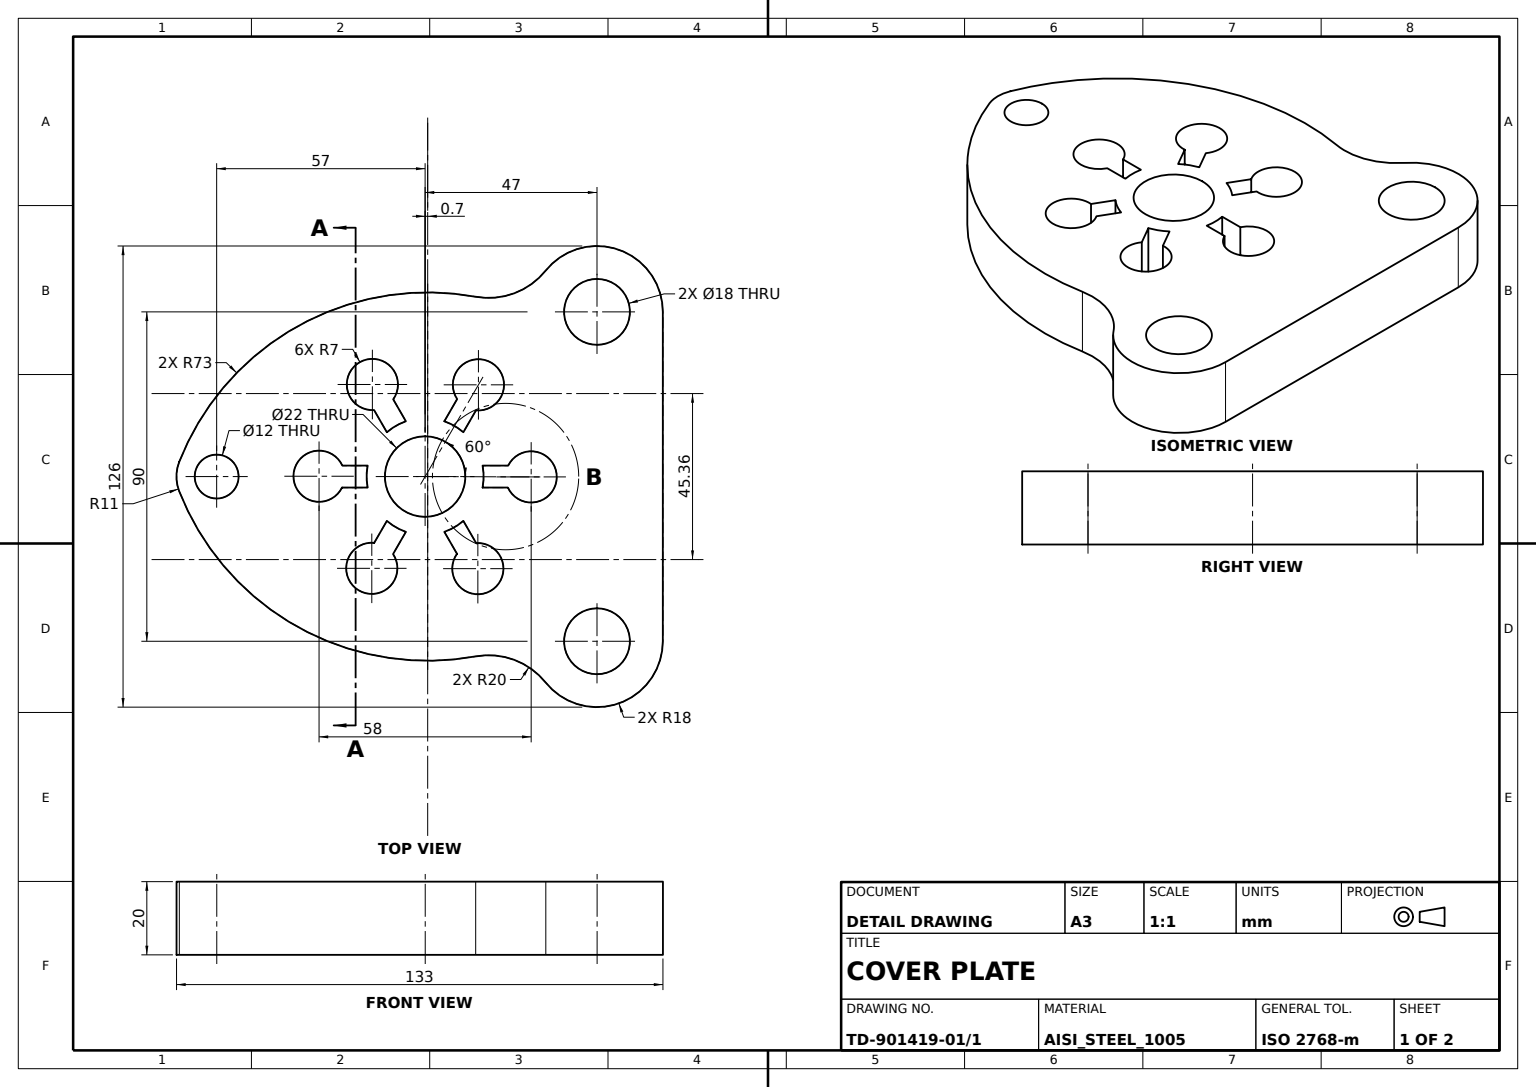
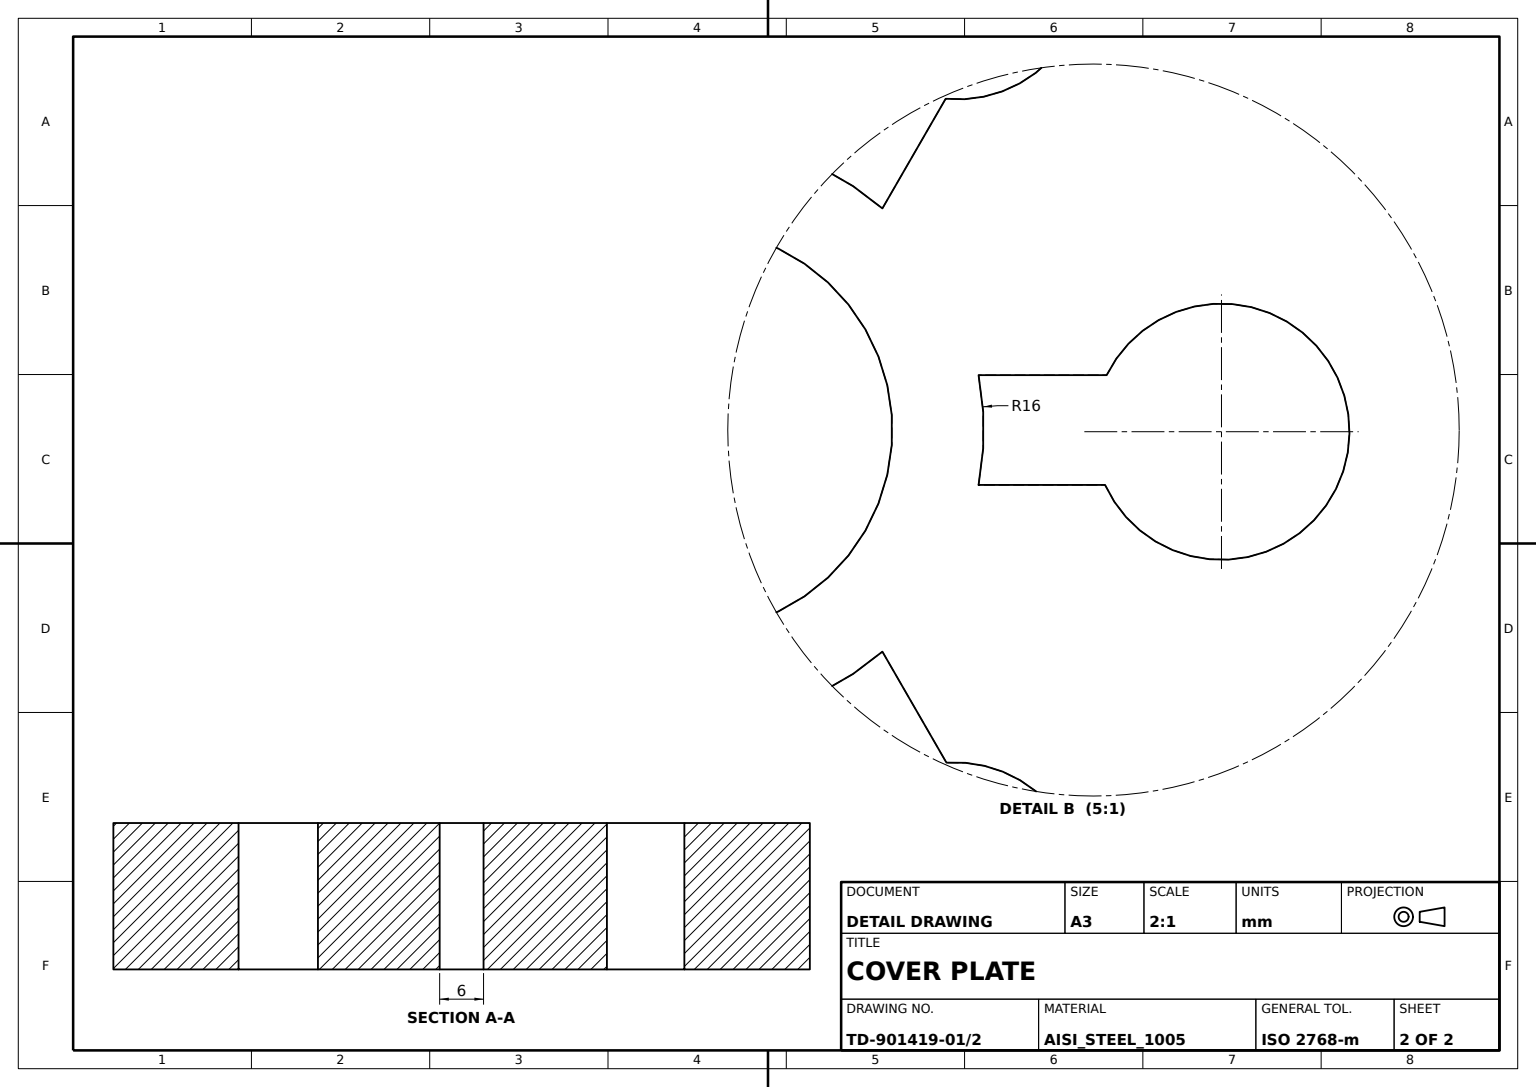
ISO-10303-21;
HEADER;
FILE_DESCRIPTION((''),'2;1');
FILE_NAME('','',(''),(''),'','','');
FILE_SCHEMA(('AUTOMOTIVE_DESIGN'));
ENDSEC;
DATA;
#1=APPLICATION_CONTEXT('');
#2=PRODUCT_CONTEXT('',#1,'mechanical');
#3=PRODUCT('','','',(#2));
#4=PRODUCT_DEFINITION_FORMATION('','',#3);
#5=PRODUCT_DEFINITION_CONTEXT('',#1,'design');
#6=PRODUCT_DEFINITION('','',#4,#5);
#7=PRODUCT_DEFINITION_SHAPE('','',#6);
#8=(LENGTH_UNIT()NAMED_UNIT(*)SI_UNIT(.MILLI.,.METRE.));
#9=(NAMED_UNIT(*)PLANE_ANGLE_UNIT()SI_UNIT($,.RADIAN.));
#10=(NAMED_UNIT(*)SI_UNIT($,.STERADIAN.)SOLID_ANGLE_UNIT());
#11=UNCERTAINTY_MEASURE_WITH_UNIT(LENGTH_MEASURE(0.005),#8,'distance_accuracy_value','');
#12=(GEOMETRIC_REPRESENTATION_CONTEXT(3)GLOBAL_UNCERTAINTY_ASSIGNED_CONTEXT((#11))GLOBAL_UNIT_ASSIGNED_CONTEXT((#8,#9,#10))REPRESENTATION_CONTEXT('',''));
#13=CARTESIAN_POINT('',(-15.716234,3.,20.));
#14=VERTEX_POINT('',#13);
#15=CARTESIAN_POINT('',(-15.716234,3.,0.));
#16=VERTEX_POINT('',#15);
#17=DIRECTION('',(0.,0.,-1.));
#18=VECTOR('',#17,1000.);
#19=LINE('',#13,#18);
#20=EDGE_CURVE('',#14,#16,#19,.T.);
#21=ORIENTED_EDGE('',*,*,#20,.T.);
#22=CARTESIAN_POINT('',(-15.716234,-3.,0.));
#23=VERTEX_POINT('',#22);
#24=CARTESIAN_POINT('',(0.,0.,0.));
#25=DIRECTION('',(0.,0.,1.));
#26=DIRECTION('',(0.,1.,0.));
#27=AXIS2_PLACEMENT_3D('',#24,#25,#26);
#28=CIRCLE('',#27,16.);
#29=EDGE_CURVE('',#16,#23,#28,.T.);
#30=ORIENTED_EDGE('',*,*,#29,.T.);
#31=CARTESIAN_POINT('',(-15.716234,-3.,20.));
#32=VERTEX_POINT('',#31);
#33=LINE('',#31,#18);
#34=EDGE_CURVE('',#32,#23,#33,.T.);
#35=ORIENTED_EDGE('',*,*,#34,.F.);
#36=CARTESIAN_POINT('',(0.,0.,20.));
#37=AXIS2_PLACEMENT_3D('',#36,#25,#26);
#38=CIRCLE('',#37,16.);
#39=EDGE_CURVE('',#14,#32,#38,.T.);
#40=ORIENTED_EDGE('',*,*,#39,.F.);
#41=EDGE_LOOP('',(#21,#30,#35,#40));
#42=FACE_BOUND('',#41,.T.);
#43=DIRECTION('',(-1.,0.,0.));
#44=AXIS2_PLACEMENT_3D('',#36,#17,#43);
#45=CYLINDRICAL_SURFACE('',#44,16.);
#46=ADVANCED_FACE('',(#42),#45,.T.);
#47=CARTESIAN_POINT('',(-67.237604,-4.023861,20.));
#48=VERTEX_POINT('',#47);
#49=CARTESIAN_POINT('',(-67.237604,-4.023861,0.));
#50=VERTEX_POINT('',#49);
#51=LINE('',#47,#18);
#52=EDGE_CURVE('',#48,#50,#51,.T.);
#53=ORIENTED_EDGE('',*,*,#52,.T.);
#54=CARTESIAN_POINT('',(13.797922,-49.135927,0.));
#55=VERTEX_POINT('',#54);
#56=CARTESIAN_POINT('',(0.702861,22.679944,0.));
#57=DIRECTION('',(0.,-1.,0.));
#58=AXIS2_PLACEMENT_3D('',#56,#25,#57);
#59=CIRCLE('',#58,73.);
#60=EDGE_CURVE('',#50,#55,#59,.T.);
#61=ORIENTED_EDGE('',*,*,#60,.T.);
#62=CARTESIAN_POINT('',(13.797922,-49.135927,20.));
#63=VERTEX_POINT('',#62);
#64=LINE('',#62,#18);
#65=EDGE_CURVE('',#63,#55,#64,.T.);
#66=ORIENTED_EDGE('',*,*,#65,.F.);
#67=CARTESIAN_POINT('',(0.702861,22.679944,20.));
#68=AXIS2_PLACEMENT_3D('',#67,#25,#57);
#69=CIRCLE('',#68,73.);
#70=EDGE_CURVE('',#48,#63,#69,.T.);
#71=ORIENTED_EDGE('',*,*,#70,.F.);
#72=EDGE_LOOP('',(#53,#61,#66,#71));
#73=FACE_BOUND('',#72,.T.);
#74=AXIS2_PLACEMENT_3D('',#67,#17,#43);
#75=CYLINDRICAL_SURFACE('',#74,73.);
#76=ADVANCED_FACE('',(#73),#75,.T.);
#77=CARTESIAN_POINT('',(-22.719384,-3.,20.));
#78=VERTEX_POINT('',#77);
#79=CARTESIAN_POINT('',(-22.632831,3.,20.));
#80=VERTEX_POINT('',#79);
#81=CARTESIAN_POINT('',(-28.999857,0.091223,20.));
#82=AXIS2_PLACEMENT_3D('',#81,#17,#26);
#83=CIRCLE('',#82,7.);
#84=EDGE_CURVE('',#78,#80,#83,.T.);
#85=ORIENTED_EDGE('',*,*,#84,.F.);
#86=CARTESIAN_POINT('',(-22.719384,-3.,0.));
#87=VERTEX_POINT('',#86);
#88=LINE('',#77,#18);
#89=EDGE_CURVE('',#78,#87,#88,.T.);
#90=ORIENTED_EDGE('',*,*,#89,.T.);
#91=CARTESIAN_POINT('',(-22.632831,3.,0.));
#92=VERTEX_POINT('',#91);
#93=CARTESIAN_POINT('',(-28.999857,0.091223,0.));
#94=AXIS2_PLACEMENT_3D('',#93,#17,#26);
#95=CIRCLE('',#94,7.);
#96=EDGE_CURVE('',#87,#92,#95,.T.);
#97=ORIENTED_EDGE('',*,*,#96,.T.);
#98=LINE('',#79,#18);
#99=EDGE_CURVE('',#80,#92,#98,.T.);
#100=ORIENTED_EDGE('',*,*,#99,.F.);
#101=EDGE_LOOP('',(#85,#90,#97,#100));
#102=FACE_BOUND('',#101,.T.);
#103=AXIS2_PLACEMENT_3D('',#81,#17,#43);
#104=CYLINDRICAL_SURFACE('',#103,7.);
#105=ADVANCED_FACE('',(#102),#104,.F.);
#106=CARTESIAN_POINT('',(13.957768,-18.175563,20.));
#107=VERTEX_POINT('',#106);
#108=CARTESIAN_POINT('',(8.718339,-21.100606,20.));
#109=VERTEX_POINT('',#108);
#110=CARTESIAN_POINT('',(14.420927,-25.160224,20.));
#111=DIRECTION('',(-0.866025404,-0.5,0.));
#112=AXIS2_PLACEMENT_3D('',#110,#17,#111);
#113=CIRCLE('',#112,7.);
#114=EDGE_CURVE('',#107,#109,#113,.T.);
#115=ORIENTED_EDGE('',*,*,#114,.F.);
#116=CARTESIAN_POINT('',(13.957768,-18.175563,0.));
#117=VERTEX_POINT('',#116);
#118=LINE('',#106,#18);
#119=EDGE_CURVE('',#107,#117,#118,.T.);
#120=ORIENTED_EDGE('',*,*,#119,.T.);
#121=CARTESIAN_POINT('',(8.718339,-21.100606,0.));
#122=VERTEX_POINT('',#121);
#123=CARTESIAN_POINT('',(14.420927,-25.160224,0.));
#124=AXIS2_PLACEMENT_3D('',#123,#17,#111);
#125=CIRCLE('',#124,7.);
#126=EDGE_CURVE('',#117,#122,#125,.T.);
#127=ORIENTED_EDGE('',*,*,#126,.T.);
#128=LINE('',#108,#18);
#129=EDGE_CURVE('',#109,#122,#128,.T.);
#130=ORIENTED_EDGE('',*,*,#129,.F.);
#131=EDGE_LOOP('',(#115,#120,#127,#130));
#132=FACE_BOUND('',#131,.T.);
#133=AXIS2_PLACEMENT_3D('',#110,#17,#43);
#134=CYLINDRICAL_SURFACE('',#133,7.);
#135=ADVANCED_FACE('',(#132),#134,.F.);
#136=CARTESIAN_POINT('',(-57.,6.,0.));
#137=VERTEX_POINT('',#136);
#138=CARTESIAN_POINT('',(-57.,0.,0.));
#139=AXIS2_PLACEMENT_3D('',#138,#25,#26);
#140=CIRCLE('',#139,6.);
#141=EDGE_CURVE('',#137,#137,#140,.T.);
#142=ORIENTED_EDGE('',*,*,#141,.T.);
#143=EDGE_LOOP('',(#142));
#144=FACE_BOUND('',#143,.T.);
#145=CARTESIAN_POINT('',(-13.914492,-18.100606,0.));
#146=VERTEX_POINT('',#145);
#147=CARTESIAN_POINT('',(-10.456193,-12.110658,0.));
#148=VERTEX_POINT('',#147);
#149=DIRECTION('',(0.5,0.866025404,0.));
#150=VECTOR('',#149,1000.);
#151=LINE('',#145,#150);
#152=EDGE_CURVE('',#146,#148,#151,.T.);
#153=ORIENTED_EDGE('',*,*,#152,.F.);
#154=CARTESIAN_POINT('',(-8.761616,-21.175563,0.));
#155=VERTEX_POINT('',#154);
#156=CARTESIAN_POINT('',(-14.57893,-25.069001,0.));
#157=DIRECTION('',(-0.866025404,0.5,0.));
#158=AXIS2_PLACEMENT_3D('',#156,#17,#157);
#159=CIRCLE('',#158,7.);
#160=EDGE_CURVE('',#155,#146,#159,.T.);
#161=ORIENTED_EDGE('',*,*,#160,.F.);
#162=CARTESIAN_POINT('',(-5.260041,-15.110658,0.));
#163=VERTEX_POINT('',#162);
#164=DIRECTION('',(-0.5,-0.866025404,0.));
#165=VECTOR('',#164,1000.);
#166=LINE('',#162,#165);
#167=EDGE_CURVE('',#163,#155,#166,.T.);
#168=ORIENTED_EDGE('',*,*,#167,.F.);
#169=AXIS2_PLACEMENT_3D('',#24,#25,#157);
#170=CIRCLE('',#169,16.);
#171=EDGE_CURVE('',#148,#163,#170,.T.);
#172=ORIENTED_EDGE('',*,*,#171,.F.);
#173=EDGE_LOOP('',(#153,#161,#168,#172));
#174=FACE_BOUND('',#173,.T.);
#175=CARTESIAN_POINT('',(47.,54.,0.));
#176=VERTEX_POINT('',#175);
#177=CARTESIAN_POINT('',(47.,45.,0.));
#178=AXIS2_PLACEMENT_3D('',#177,#25,#26);
#179=CIRCLE('',#178,9.);
#180=EDGE_CURVE('',#176,#176,#179,.T.);
#181=ORIENTED_EDGE('',*,*,#180,.T.);
#182=EDGE_LOOP('',(#181));
#183=FACE_BOUND('',#182,.T.);
#184=CARTESIAN_POINT('',(22.719384,3.,0.));
#185=VERTEX_POINT('',#184);
#186=CARTESIAN_POINT('',(22.632831,-3.,0.));
#187=VERTEX_POINT('',#186);
#188=CARTESIAN_POINT('',(28.999857,-0.091223,0.));
#189=AXIS2_PLACEMENT_3D('',#188,#17,#57);
#190=CIRCLE('',#189,7.);
#191=EDGE_CURVE('',#185,#187,#190,.T.);
#192=ORIENTED_EDGE('',*,*,#191,.F.);
#193=CARTESIAN_POINT('',(15.716234,3.,0.));
#194=VERTEX_POINT('',#193);
#195=DIRECTION('',(1.,0.,0.));
#196=VECTOR('',#195,1000.);
#197=LINE('',#193,#196);
#198=EDGE_CURVE('',#194,#185,#197,.T.);
#199=ORIENTED_EDGE('',*,*,#198,.F.);
#200=CARTESIAN_POINT('',(15.716234,-3.,0.));
#201=VERTEX_POINT('',#200);
#202=AXIS2_PLACEMENT_3D('',#24,#25,#57);
#203=CIRCLE('',#202,16.);
#204=EDGE_CURVE('',#201,#194,#203,.T.);
#205=ORIENTED_EDGE('',*,*,#204,.F.);
#206=VECTOR('',#43,1000.);
#207=LINE('',#186,#206);
#208=EDGE_CURVE('',#187,#201,#207,.T.);
#209=ORIENTED_EDGE('',*,*,#208,.F.);
#210=EDGE_LOOP('',(#192,#199,#205,#209));
#211=FACE_BOUND('',#210,.T.);
#212=CARTESIAN_POINT('',(5.260041,-15.110658,0.));
#213=VERTEX_POINT('',#212);
#214=CARTESIAN_POINT('',(10.456193,-12.110658,0.));
#215=VERTEX_POINT('',#214);
#216=AXIS2_PLACEMENT_3D('',#24,#25,#111);
#217=CIRCLE('',#216,16.);
#218=EDGE_CURVE('',#213,#215,#217,.T.);
#219=ORIENTED_EDGE('',*,*,#218,.F.);
#220=DIRECTION('',(-0.5,0.866025404,0.));
#221=VECTOR('',#220,1000.);
#222=LINE('',#121,#221);
#223=EDGE_CURVE('',#122,#213,#222,.T.);
#224=ORIENTED_EDGE('',*,*,#223,.F.);
#225=ORIENTED_EDGE('',*,*,#126,.F.);
#226=DIRECTION('',(0.5,-0.866025404,0.));
#227=VECTOR('',#226,1000.);
#228=LINE('',#214,#227);
#229=EDGE_CURVE('',#215,#117,#228,.T.);
#230=ORIENTED_EDGE('',*,*,#229,.F.);
#231=EDGE_LOOP('',(#219,#224,#225,#230));
#232=FACE_BOUND('',#231,.T.);
#233=CARTESIAN_POINT('',(0.,11.,0.));
#234=VERTEX_POINT('',#233);
#235=CIRCLE('',#27,11.);
#236=EDGE_CURVE('',#234,#234,#235,.T.);
#237=ORIENTED_EDGE('',*,*,#236,.T.);
#238=EDGE_LOOP('',(#237));
#239=FACE_BOUND('',#238,.T.);
#240=LINE('',#22,#206);
#241=EDGE_CURVE('',#23,#87,#240,.T.);
#242=ORIENTED_EDGE('',*,*,#241,.F.);
#243=ORIENTED_EDGE('',*,*,#29,.F.);
#244=LINE('',#91,#196);
#245=EDGE_CURVE('',#92,#16,#244,.T.);
#246=ORIENTED_EDGE('',*,*,#245,.F.);
#247=ORIENTED_EDGE('',*,*,#96,.F.);
#248=EDGE_LOOP('',(#242,#243,#246,#247));
#249=FACE_BOUND('',#248,.T.);
#250=ORIENTED_EDGE('',*,*,#60,.F.);
#251=CARTESIAN_POINT('',(-67.237604,4.023861,0.));
#252=VERTEX_POINT('',#251);
#253=CIRCLE('',#139,11.);
#254=EDGE_CURVE('',#252,#50,#253,.T.);
#255=ORIENTED_EDGE('',*,*,#254,.F.);
#256=CARTESIAN_POINT('',(13.797922,49.135927,0.));
#257=VERTEX_POINT('',#256);
#258=CARTESIAN_POINT('',(0.702861,-22.679944,0.));
#259=AXIS2_PLACEMENT_3D('',#258,#25,#26);
#260=CIRCLE('',#259,73.);
#261=EDGE_CURVE('',#257,#252,#260,.T.);
#262=ORIENTED_EDGE('',*,*,#261,.F.);
#263=CARTESIAN_POINT('',(32.972131,56.279135,0.));
#264=VERTEX_POINT('',#263);
#265=CARTESIAN_POINT('',(17.38561,68.811508,0.));
#266=AXIS2_PLACEMENT_3D('',#265,#17,#26);
#267=CIRCLE('',#266,20.);
#268=EDGE_CURVE('',#264,#257,#267,.T.);
#269=ORIENTED_EDGE('',*,*,#268,.F.);
#270=CARTESIAN_POINT('',(65.,45.,0.));
#271=VERTEX_POINT('',#270);
#272=CIRCLE('',#178,18.);
#273=EDGE_CURVE('',#271,#264,#272,.T.);
#274=ORIENTED_EDGE('',*,*,#273,.F.);
#275=CARTESIAN_POINT('',(65.,-45.,0.));
#276=VERTEX_POINT('',#275);
#277=VECTOR('',#26,1000.);
#278=LINE('',#275,#277);
#279=EDGE_CURVE('',#276,#271,#278,.T.);
#280=ORIENTED_EDGE('',*,*,#279,.F.);
#281=CARTESIAN_POINT('',(32.972131,-56.279135,0.));
#282=VERTEX_POINT('',#281);
#283=CARTESIAN_POINT('',(47.,-45.,0.));
#284=AXIS2_PLACEMENT_3D('',#283,#25,#26);
#285=CIRCLE('',#284,18.);
#286=EDGE_CURVE('',#282,#276,#285,.T.);
#287=ORIENTED_EDGE('',*,*,#286,.F.);
#288=CARTESIAN_POINT('',(17.38561,-68.811508,0.));
#289=AXIS2_PLACEMENT_3D('',#288,#17,#57);
#290=CIRCLE('',#289,20.);
#291=EDGE_CURVE('',#55,#282,#290,.T.);
#292=ORIENTED_EDGE('',*,*,#291,.F.);
#293=EDGE_LOOP('',(#250,#255,#262,#269,#274,#280,#287,#292));
#294=FACE_BOUND('',#293,.T.);
#295=CARTESIAN_POINT('',(47.,-36.,0.));
#296=VERTEX_POINT('',#295);
#297=CIRCLE('',#284,9.);
#298=EDGE_CURVE('',#296,#296,#297,.T.);
#299=ORIENTED_EDGE('',*,*,#298,.T.);
#300=EDGE_LOOP('',(#299));
#301=FACE_BOUND('',#300,.T.);
#302=CARTESIAN_POINT('',(10.456193,12.110658,0.));
#303=VERTEX_POINT('',#302);
#304=CARTESIAN_POINT('',(5.260041,15.110658,0.));
#305=VERTEX_POINT('',#304);
#306=DIRECTION('',(0.866025404,-0.5,0.));
#307=AXIS2_PLACEMENT_3D('',#24,#25,#306);
#308=CIRCLE('',#307,16.);
#309=EDGE_CURVE('',#303,#305,#308,.T.);
#310=ORIENTED_EDGE('',*,*,#309,.F.);
#311=CARTESIAN_POINT('',(13.914492,18.100606,0.));
#312=VERTEX_POINT('',#311);
#313=LINE('',#311,#165);
#314=EDGE_CURVE('',#312,#303,#313,.T.);
#315=ORIENTED_EDGE('',*,*,#314,.F.);
#316=CARTESIAN_POINT('',(8.761616,21.175563,0.));
#317=VERTEX_POINT('',#316);
#318=CARTESIAN_POINT('',(14.57893,25.069001,0.));
#319=AXIS2_PLACEMENT_3D('',#318,#17,#306);
#320=CIRCLE('',#319,7.);
#321=EDGE_CURVE('',#317,#312,#320,.T.);
#322=ORIENTED_EDGE('',*,*,#321,.F.);
#323=LINE('',#304,#150);
#324=EDGE_CURVE('',#305,#317,#323,.T.);
#325=ORIENTED_EDGE('',*,*,#324,.F.);
#326=EDGE_LOOP('',(#310,#315,#322,#325));
#327=FACE_BOUND('',#326,.T.);
#328=CARTESIAN_POINT('',(-5.260041,15.110658,0.));
#329=VERTEX_POINT('',#328);
#330=CARTESIAN_POINT('',(-10.456193,12.110658,0.));
#331=VERTEX_POINT('',#330);
#332=DIRECTION('',(0.866025404,0.5,0.));
#333=AXIS2_PLACEMENT_3D('',#24,#25,#332);
#334=CIRCLE('',#333,16.);
#335=EDGE_CURVE('',#329,#331,#334,.T.);
#336=ORIENTED_EDGE('',*,*,#335,.F.);
#337=CARTESIAN_POINT('',(-8.718339,21.100606,0.));
#338=VERTEX_POINT('',#337);
#339=LINE('',#337,#227);
#340=EDGE_CURVE('',#338,#329,#339,.T.);
#341=ORIENTED_EDGE('',*,*,#340,.F.);
#342=CARTESIAN_POINT('',(-13.957768,18.175563,0.));
#343=VERTEX_POINT('',#342);
#344=CARTESIAN_POINT('',(-14.420927,25.160224,0.));
#345=AXIS2_PLACEMENT_3D('',#344,#17,#332);
#346=CIRCLE('',#345,7.);
#347=EDGE_CURVE('',#343,#338,#346,.T.);
#348=ORIENTED_EDGE('',*,*,#347,.F.);
#349=LINE('',#330,#221);
#350=EDGE_CURVE('',#331,#343,#349,.T.);
#351=ORIENTED_EDGE('',*,*,#350,.F.);
#352=EDGE_LOOP('',(#336,#341,#348,#351));
#353=FACE_BOUND('',#352,.T.);
#354=AXIS2_PLACEMENT_3D('',#138,#25,#195);
#355=PLANE('',#354);
#356=ADVANCED_FACE('',(#144,#174,#183,#211,#232,#239,#249,#294,#301,#327,#353),#355,.F.);
#357=CARTESIAN_POINT('',(-5.260041,15.110658,20.));
#358=VERTEX_POINT('',#357);
#359=CARTESIAN_POINT('',(-10.456193,12.110658,20.));
#360=VERTEX_POINT('',#359);
#361=AXIS2_PLACEMENT_3D('',#36,#25,#332);
#362=CIRCLE('',#361,16.);
#363=EDGE_CURVE('',#358,#360,#362,.T.);
#364=ORIENTED_EDGE('',*,*,#363,.F.);
#365=LINE('',#357,#18);
#366=EDGE_CURVE('',#358,#329,#365,.T.);
#367=ORIENTED_EDGE('',*,*,#366,.T.);
#368=ORIENTED_EDGE('',*,*,#335,.T.);
#369=LINE('',#359,#18);
#370=EDGE_CURVE('',#360,#331,#369,.T.);
#371=ORIENTED_EDGE('',*,*,#370,.F.);
#372=EDGE_LOOP('',(#364,#367,#368,#371));
#373=FACE_BOUND('',#372,.T.);
#374=ADVANCED_FACE('',(#373),#45,.T.);
#375=CARTESIAN_POINT('',(15.716234,3.,20.));
#376=VERTEX_POINT('',#375);
#377=CARTESIAN_POINT('',(22.719384,3.,20.));
#378=VERTEX_POINT('',#377);
#379=LINE('',#375,#196);
#380=EDGE_CURVE('',#376,#378,#379,.T.);
#381=ORIENTED_EDGE('',*,*,#380,.F.);
#382=LINE('',#375,#18);
#383=EDGE_CURVE('',#376,#194,#382,.T.);
#384=ORIENTED_EDGE('',*,*,#383,.T.);
#385=ORIENTED_EDGE('',*,*,#198,.T.);
#386=LINE('',#377,#18);
#387=EDGE_CURVE('',#378,#185,#386,.T.);
#388=ORIENTED_EDGE('',*,*,#387,.F.);
#389=EDGE_LOOP('',(#381,#384,#385,#388));
#390=FACE_BOUND('',#389,.T.);
#391=AXIS2_PLACEMENT_3D('',#375,#26,#43);
#392=PLANE('',#391);
#393=ADVANCED_FACE('',(#390),#392,.F.);
#394=CARTESIAN_POINT('',(-8.718339,21.100606,20.));
#395=VERTEX_POINT('',#394);
#396=LINE('',#394,#18);
#397=EDGE_CURVE('',#395,#338,#396,.T.);
#398=ORIENTED_EDGE('',*,*,#397,.F.);
#399=CARTESIAN_POINT('',(-13.957768,18.175563,20.));
#400=VERTEX_POINT('',#399);
#401=CARTESIAN_POINT('',(-14.420927,25.160224,20.));
#402=AXIS2_PLACEMENT_3D('',#401,#17,#332);
#403=CIRCLE('',#402,7.);
#404=EDGE_CURVE('',#400,#395,#403,.T.);
#405=ORIENTED_EDGE('',*,*,#404,.F.);
#406=LINE('',#399,#18);
#407=EDGE_CURVE('',#400,#343,#406,.T.);
#408=ORIENTED_EDGE('',*,*,#407,.T.);
#409=ORIENTED_EDGE('',*,*,#347,.T.);
#410=EDGE_LOOP('',(#398,#405,#408,#409));
#411=FACE_BOUND('',#410,.T.);
#412=AXIS2_PLACEMENT_3D('',#401,#17,#43);
#413=CYLINDRICAL_SURFACE('',#412,7.);
#414=ADVANCED_FACE('',(#411),#413,.F.);
#415=CARTESIAN_POINT('',(47.,54.,20.));
#416=VERTEX_POINT('',#415);
#417=CARTESIAN_POINT('',(47.,45.,20.));
#418=AXIS2_PLACEMENT_3D('',#417,#25,#26);
#419=CIRCLE('',#418,9.);
#420=EDGE_CURVE('',#416,#416,#419,.T.);
#421=ORIENTED_EDGE('',*,*,#420,.F.);
#422=EDGE_LOOP('',(#421));
#423=FACE_BOUND('',#422,.T.);
#424=ORIENTED_EDGE('',*,*,#114,.T.);
#425=CARTESIAN_POINT('',(5.260041,-15.110658,20.));
#426=VERTEX_POINT('',#425);
#427=LINE('',#108,#221);
#428=EDGE_CURVE('',#109,#426,#427,.T.);
#429=ORIENTED_EDGE('',*,*,#428,.T.);
#430=CARTESIAN_POINT('',(10.456193,-12.110658,20.));
#431=VERTEX_POINT('',#430);
#432=AXIS2_PLACEMENT_3D('',#36,#25,#111);
#433=CIRCLE('',#432,16.);
#434=EDGE_CURVE('',#426,#431,#433,.T.);
#435=ORIENTED_EDGE('',*,*,#434,.T.);
#436=LINE('',#430,#227);
#437=EDGE_CURVE('',#431,#107,#436,.T.);
#438=ORIENTED_EDGE('',*,*,#437,.T.);
#439=EDGE_LOOP('',(#424,#429,#435,#438));
#440=FACE_BOUND('',#439,.T.);
#441=CARTESIAN_POINT('',(5.260041,15.110658,20.));
#442=VERTEX_POINT('',#441);
#443=CARTESIAN_POINT('',(8.761616,21.175563,20.));
#444=VERTEX_POINT('',#443);
#445=LINE('',#441,#150);
#446=EDGE_CURVE('',#442,#444,#445,.T.);
#447=ORIENTED_EDGE('',*,*,#446,.T.);
#448=CARTESIAN_POINT('',(13.914492,18.100606,20.));
#449=VERTEX_POINT('',#448);
#450=CARTESIAN_POINT('',(14.57893,25.069001,20.));
#451=AXIS2_PLACEMENT_3D('',#450,#17,#306);
#452=CIRCLE('',#451,7.);
#453=EDGE_CURVE('',#444,#449,#452,.T.);
#454=ORIENTED_EDGE('',*,*,#453,.T.);
#455=CARTESIAN_POINT('',(10.456193,12.110658,20.));
#456=VERTEX_POINT('',#455);
#457=LINE('',#448,#165);
#458=EDGE_CURVE('',#449,#456,#457,.T.);
#459=ORIENTED_EDGE('',*,*,#458,.T.);
#460=AXIS2_PLACEMENT_3D('',#36,#25,#306);
#461=CIRCLE('',#460,16.);
#462=EDGE_CURVE('',#456,#442,#461,.T.);
#463=ORIENTED_EDGE('',*,*,#462,.T.);
#464=EDGE_LOOP('',(#447,#454,#459,#463));
#465=FACE_BOUND('',#464,.T.);
#466=LINE('',#31,#206);
#467=EDGE_CURVE('',#32,#78,#466,.T.);
#468=ORIENTED_EDGE('',*,*,#467,.T.);
#469=ORIENTED_EDGE('',*,*,#84,.T.);
#470=LINE('',#79,#196);
#471=EDGE_CURVE('',#80,#14,#470,.T.);
#472=ORIENTED_EDGE('',*,*,#471,.T.);
#473=ORIENTED_EDGE('',*,*,#39,.T.);
#474=EDGE_LOOP('',(#468,#469,#472,#473));
#475=FACE_BOUND('',#474,.T.);
#476=CARTESIAN_POINT('',(32.972131,-56.279135,20.));
#477=VERTEX_POINT('',#476);
#478=CARTESIAN_POINT('',(17.38561,-68.811508,20.));
#479=AXIS2_PLACEMENT_3D('',#478,#17,#57);
#480=CIRCLE('',#479,20.);
#481=EDGE_CURVE('',#63,#477,#480,.T.);
#482=ORIENTED_EDGE('',*,*,#481,.T.);
#483=CARTESIAN_POINT('',(65.,-45.,20.));
#484=VERTEX_POINT('',#483);
#485=CARTESIAN_POINT('',(47.,-45.,20.));
#486=AXIS2_PLACEMENT_3D('',#485,#25,#26);
#487=CIRCLE('',#486,18.);
#488=EDGE_CURVE('',#477,#484,#487,.T.);
#489=ORIENTED_EDGE('',*,*,#488,.T.);
#490=CARTESIAN_POINT('',(65.,45.,20.));
#491=VERTEX_POINT('',#490);
#492=LINE('',#483,#277);
#493=EDGE_CURVE('',#484,#491,#492,.T.);
#494=ORIENTED_EDGE('',*,*,#493,.T.);
#495=CARTESIAN_POINT('',(32.972131,56.279135,20.));
#496=VERTEX_POINT('',#495);
#497=CIRCLE('',#418,18.);
#498=EDGE_CURVE('',#491,#496,#497,.T.);
#499=ORIENTED_EDGE('',*,*,#498,.T.);
#500=CARTESIAN_POINT('',(13.797922,49.135927,20.));
#501=VERTEX_POINT('',#500);
#502=CARTESIAN_POINT('',(17.38561,68.811508,20.));
#503=AXIS2_PLACEMENT_3D('',#502,#17,#26);
#504=CIRCLE('',#503,20.);
#505=EDGE_CURVE('',#496,#501,#504,.T.);
#506=ORIENTED_EDGE('',*,*,#505,.T.);
#507=CARTESIAN_POINT('',(-67.237604,4.023861,20.));
#508=VERTEX_POINT('',#507);
#509=CARTESIAN_POINT('',(0.702861,-22.679944,20.));
#510=AXIS2_PLACEMENT_3D('',#509,#25,#26);
#511=CIRCLE('',#510,73.);
#512=EDGE_CURVE('',#501,#508,#511,.T.);
#513=ORIENTED_EDGE('',*,*,#512,.T.);
#514=CARTESIAN_POINT('',(-57.,0.,20.));
#515=AXIS2_PLACEMENT_3D('',#514,#25,#26);
#516=CIRCLE('',#515,11.);
#517=EDGE_CURVE('',#508,#48,#516,.T.);
#518=ORIENTED_EDGE('',*,*,#517,.T.);
#519=ORIENTED_EDGE('',*,*,#70,.T.);
#520=EDGE_LOOP('',(#482,#489,#494,#499,#506,#513,#518,#519));
#521=FACE_BOUND('',#520,.T.);
#522=CARTESIAN_POINT('',(-57.,6.,20.));
#523=VERTEX_POINT('',#522);
#524=CIRCLE('',#515,6.);
#525=EDGE_CURVE('',#523,#523,#524,.T.);
#526=ORIENTED_EDGE('',*,*,#525,.F.);
#527=EDGE_LOOP('',(#526));
#528=FACE_BOUND('',#527,.T.);
#529=LINE('',#359,#221);
#530=EDGE_CURVE('',#360,#400,#529,.T.);
#531=ORIENTED_EDGE('',*,*,#530,.T.);
#532=ORIENTED_EDGE('',*,*,#404,.T.);
#533=LINE('',#394,#227);
#534=EDGE_CURVE('',#395,#358,#533,.T.);
#535=ORIENTED_EDGE('',*,*,#534,.T.);
#536=ORIENTED_EDGE('',*,*,#363,.T.);
#537=EDGE_LOOP('',(#531,#532,#535,#536));
#538=FACE_BOUND('',#537,.T.);
#539=CARTESIAN_POINT('',(-5.260041,-15.110658,20.));
#540=VERTEX_POINT('',#539);
#541=CARTESIAN_POINT('',(-8.761616,-21.175563,20.));
#542=VERTEX_POINT('',#541);
#543=LINE('',#539,#165);
#544=EDGE_CURVE('',#540,#542,#543,.T.);
#545=ORIENTED_EDGE('',*,*,#544,.T.);
#546=CARTESIAN_POINT('',(-13.914492,-18.100606,20.));
#547=VERTEX_POINT('',#546);
#548=CARTESIAN_POINT('',(-14.57893,-25.069001,20.));
#549=AXIS2_PLACEMENT_3D('',#548,#17,#157);
#550=CIRCLE('',#549,7.);
#551=EDGE_CURVE('',#542,#547,#550,.T.);
#552=ORIENTED_EDGE('',*,*,#551,.T.);
#553=CARTESIAN_POINT('',(-10.456193,-12.110658,20.));
#554=VERTEX_POINT('',#553);
#555=LINE('',#546,#150);
#556=EDGE_CURVE('',#547,#554,#555,.T.);
#557=ORIENTED_EDGE('',*,*,#556,.T.);
#558=AXIS2_PLACEMENT_3D('',#36,#25,#157);
#559=CIRCLE('',#558,16.);
#560=EDGE_CURVE('',#554,#540,#559,.T.);
#561=ORIENTED_EDGE('',*,*,#560,.T.);
#562=EDGE_LOOP('',(#545,#552,#557,#561));
#563=FACE_BOUND('',#562,.T.);
#564=CARTESIAN_POINT('',(0.,11.,20.));
#565=VERTEX_POINT('',#564);
#566=CIRCLE('',#37,11.);
#567=EDGE_CURVE('',#565,#565,#566,.T.);
#568=ORIENTED_EDGE('',*,*,#567,.F.);
#569=EDGE_LOOP('',(#568));
#570=FACE_BOUND('',#569,.T.);
#571=CARTESIAN_POINT('',(22.632831,-3.,20.));
#572=VERTEX_POINT('',#571);
#573=CARTESIAN_POINT('',(28.999857,-0.091223,20.));
#574=AXIS2_PLACEMENT_3D('',#573,#17,#57);
#575=CIRCLE('',#574,7.);
#576=EDGE_CURVE('',#378,#572,#575,.T.);
#577=ORIENTED_EDGE('',*,*,#576,.T.);
#578=CARTESIAN_POINT('',(15.716234,-3.,20.));
#579=VERTEX_POINT('',#578);
#580=LINE('',#571,#206);
#581=EDGE_CURVE('',#572,#579,#580,.T.);
#582=ORIENTED_EDGE('',*,*,#581,.T.);
#583=AXIS2_PLACEMENT_3D('',#36,#25,#57);
#584=CIRCLE('',#583,16.);
#585=EDGE_CURVE('',#579,#376,#584,.T.);
#586=ORIENTED_EDGE('',*,*,#585,.T.);
#587=ORIENTED_EDGE('',*,*,#380,.T.);
#588=EDGE_LOOP('',(#577,#582,#586,#587));
#589=FACE_BOUND('',#588,.T.);
#590=CARTESIAN_POINT('',(47.,-36.,20.));
#591=VERTEX_POINT('',#590);
#592=CIRCLE('',#486,9.);
#593=EDGE_CURVE('',#591,#591,#592,.T.);
#594=ORIENTED_EDGE('',*,*,#593,.F.);
#595=EDGE_LOOP('',(#594));
#596=FACE_BOUND('',#595,.T.);
#597=AXIS2_PLACEMENT_3D('',#514,#25,#195);
#598=PLANE('',#597);
#599=ADVANCED_FACE('',(#423,#440,#465,#475,#521,#528,#538,#563,#570,#589,#596),#598,.T.);
#600=ORIENTED_EDGE('',*,*,#481,.F.);
#601=ORIENTED_EDGE('',*,*,#65,.T.);
#602=ORIENTED_EDGE('',*,*,#291,.T.);
#603=LINE('',#476,#18);
#604=EDGE_CURVE('',#477,#282,#603,.T.);
#605=ORIENTED_EDGE('',*,*,#604,.F.);
#606=EDGE_LOOP('',(#600,#601,#602,#605));
#607=FACE_BOUND('',#606,.T.);
#608=AXIS2_PLACEMENT_3D('',#478,#17,#43);
#609=CYLINDRICAL_SURFACE('',#608,20.);
#610=ADVANCED_FACE('',(#607),#609,.F.);
#611=ORIENTED_EDGE('',*,*,#458,.F.);
#612=LINE('',#448,#18);
#613=EDGE_CURVE('',#449,#312,#612,.T.);
#614=ORIENTED_EDGE('',*,*,#613,.T.);
#615=ORIENTED_EDGE('',*,*,#314,.T.);
#616=LINE('',#455,#18);
#617=EDGE_CURVE('',#456,#303,#616,.T.);
#618=ORIENTED_EDGE('',*,*,#617,.F.);
#619=EDGE_LOOP('',(#611,#614,#615,#618));
#620=FACE_BOUND('',#619,.T.);
#621=AXIS2_PLACEMENT_3D('',#448,#306,#149);
#622=PLANE('',#621);
#623=ADVANCED_FACE('',(#620),#622,.F.);
#624=ORIENTED_EDGE('',*,*,#567,.T.);
#625=EDGE_LOOP('',(#624));
#626=FACE_BOUND('',#625,.T.);
#627=ORIENTED_EDGE('',*,*,#236,.F.);
#628=EDGE_LOOP('',(#627));
#629=FACE_BOUND('',#628,.T.);
#630=CYLINDRICAL_SURFACE('',#44,11.);
#631=ADVANCED_FACE('',(#626,#629),#630,.F.);
#632=ORIENTED_EDGE('',*,*,#534,.F.);
#633=ORIENTED_EDGE('',*,*,#397,.T.);
#634=ORIENTED_EDGE('',*,*,#340,.T.);
#635=ORIENTED_EDGE('',*,*,#366,.F.);
#636=EDGE_LOOP('',(#632,#633,#634,#635));
#637=FACE_BOUND('',#636,.T.);
#638=AXIS2_PLACEMENT_3D('',#394,#332,#220);
#639=PLANE('',#638);
#640=ADVANCED_FACE('',(#637),#639,.F.);
#641=LINE('',#495,#18);
#642=EDGE_CURVE('',#496,#264,#641,.T.);
#643=ORIENTED_EDGE('',*,*,#642,.F.);
#644=ORIENTED_EDGE('',*,*,#498,.F.);
#645=LINE('',#490,#18);
#646=EDGE_CURVE('',#491,#271,#645,.T.);
#647=ORIENTED_EDGE('',*,*,#646,.T.);
#648=ORIENTED_EDGE('',*,*,#273,.T.);
#649=EDGE_LOOP('',(#643,#644,#647,#648));
#650=FACE_BOUND('',#649,.T.);
#651=AXIS2_PLACEMENT_3D('',#417,#17,#43);
#652=CYLINDRICAL_SURFACE('',#651,18.);
#653=ADVANCED_FACE('',(#650),#652,.T.);
#654=LINE('',#539,#18);
#655=EDGE_CURVE('',#540,#163,#654,.T.);
#656=ORIENTED_EDGE('',*,*,#655,.T.);
#657=ORIENTED_EDGE('',*,*,#167,.T.);
#658=LINE('',#541,#18);
#659=EDGE_CURVE('',#542,#155,#658,.T.);
#660=ORIENTED_EDGE('',*,*,#659,.F.);
#661=ORIENTED_EDGE('',*,*,#544,.F.);
#662=EDGE_LOOP('',(#656,#657,#660,#661));
#663=FACE_BOUND('',#662,.T.);
#664=AXIS2_PLACEMENT_3D('',#539,#306,#149);
#665=PLANE('',#664);
#666=ADVANCED_FACE('',(#663),#665,.F.);
#667=LINE('',#430,#18);
#668=EDGE_CURVE('',#431,#215,#667,.T.);
#669=ORIENTED_EDGE('',*,*,#668,.T.);
#670=ORIENTED_EDGE('',*,*,#229,.T.);
#671=ORIENTED_EDGE('',*,*,#119,.F.);
#672=ORIENTED_EDGE('',*,*,#437,.F.);
#673=EDGE_LOOP('',(#669,#670,#671,#672));
#674=FACE_BOUND('',#673,.T.);
#675=AXIS2_PLACEMENT_3D('',#430,#332,#220);
#676=PLANE('',#675);
#677=ADVANCED_FACE('',(#674),#676,.F.);
#678=LINE('',#578,#18);
#679=EDGE_CURVE('',#579,#201,#678,.T.);
#680=ORIENTED_EDGE('',*,*,#679,.F.);
#681=ORIENTED_EDGE('',*,*,#581,.F.);
#682=LINE('',#571,#18);
#683=EDGE_CURVE('',#572,#187,#682,.T.);
#684=ORIENTED_EDGE('',*,*,#683,.T.);
#685=ORIENTED_EDGE('',*,*,#208,.T.);
#686=EDGE_LOOP('',(#680,#681,#684,#685));
#687=FACE_BOUND('',#686,.T.);
#688=AXIS2_PLACEMENT_3D('',#571,#57,#17);
#689=PLANE('',#688);
#690=ADVANCED_FACE('',(#687),#689,.F.);
#691=LINE('',#443,#18);
#692=EDGE_CURVE('',#444,#317,#691,.T.);
#693=ORIENTED_EDGE('',*,*,#692,.F.);
#694=ORIENTED_EDGE('',*,*,#446,.F.);
#695=LINE('',#441,#18);
#696=EDGE_CURVE('',#442,#305,#695,.T.);
#697=ORIENTED_EDGE('',*,*,#696,.T.);
#698=ORIENTED_EDGE('',*,*,#324,.T.);
#699=EDGE_LOOP('',(#693,#694,#697,#698));
#700=FACE_BOUND('',#699,.T.);
#701=AXIS2_PLACEMENT_3D('',#441,#157,#164);
#702=PLANE('',#701);
#703=ADVANCED_FACE('',(#700),#702,.F.);
#704=ORIENTED_EDGE('',*,*,#420,.T.);
#705=EDGE_LOOP('',(#704));
#706=FACE_BOUND('',#705,.T.);
#707=ORIENTED_EDGE('',*,*,#180,.F.);
#708=EDGE_LOOP('',(#707));
#709=FACE_BOUND('',#708,.T.);
#710=CYLINDRICAL_SURFACE('',#651,9.);
#711=ADVANCED_FACE('',(#706,#709),#710,.F.);
#712=ORIENTED_EDGE('',*,*,#642,.T.);
#713=ORIENTED_EDGE('',*,*,#268,.T.);
#714=LINE('',#500,#18);
#715=EDGE_CURVE('',#501,#257,#714,.T.);
#716=ORIENTED_EDGE('',*,*,#715,.F.);
#717=ORIENTED_EDGE('',*,*,#505,.F.);
#718=EDGE_LOOP('',(#712,#713,#716,#717));
#719=FACE_BOUND('',#718,.T.);
#720=AXIS2_PLACEMENT_3D('',#502,#17,#43);
#721=CYLINDRICAL_SURFACE('',#720,20.);
#722=ADVANCED_FACE('',(#719),#721,.F.);
#723=ORIENTED_EDGE('',*,*,#387,.T.);
#724=ORIENTED_EDGE('',*,*,#191,.T.);
#725=ORIENTED_EDGE('',*,*,#683,.F.);
#726=ORIENTED_EDGE('',*,*,#576,.F.);
#727=EDGE_LOOP('',(#723,#724,#725,#726));
#728=FACE_BOUND('',#727,.T.);
#729=AXIS2_PLACEMENT_3D('',#573,#17,#43);
#730=CYLINDRICAL_SURFACE('',#729,7.);
#731=ADVANCED_FACE('',(#728),#730,.F.);
#732=LINE('',#546,#18);
#733=EDGE_CURVE('',#547,#146,#732,.T.);
#734=ORIENTED_EDGE('',*,*,#733,.F.);
#735=ORIENTED_EDGE('',*,*,#551,.F.);
#736=ORIENTED_EDGE('',*,*,#659,.T.);
#737=ORIENTED_EDGE('',*,*,#160,.T.);
#738=EDGE_LOOP('',(#734,#735,#736,#737));
#739=FACE_BOUND('',#738,.T.);
#740=AXIS2_PLACEMENT_3D('',#548,#17,#43);
#741=CYLINDRICAL_SURFACE('',#740,7.);
#742=ADVANCED_FACE('',(#739),#741,.F.);
#743=ORIENTED_EDGE('',*,*,#370,.T.);
#744=ORIENTED_EDGE('',*,*,#350,.T.);
#745=ORIENTED_EDGE('',*,*,#407,.F.);
#746=ORIENTED_EDGE('',*,*,#530,.F.);
#747=EDGE_LOOP('',(#743,#744,#745,#746));
#748=FACE_BOUND('',#747,.T.);
#749=AXIS2_PLACEMENT_3D('',#359,#111,#226);
#750=PLANE('',#749);
#751=ADVANCED_FACE('',(#748),#750,.F.);
#752=ORIENTED_EDGE('',*,*,#696,.F.);
#753=ORIENTED_EDGE('',*,*,#462,.F.);
#754=ORIENTED_EDGE('',*,*,#617,.T.);
#755=ORIENTED_EDGE('',*,*,#309,.T.);
#756=EDGE_LOOP('',(#752,#753,#754,#755));
#757=FACE_BOUND('',#756,.T.);
#758=ADVANCED_FACE('',(#757),#45,.T.);
#759=ORIENTED_EDGE('',*,*,#585,.F.);
#760=ORIENTED_EDGE('',*,*,#679,.T.);
#761=ORIENTED_EDGE('',*,*,#204,.T.);
#762=ORIENTED_EDGE('',*,*,#383,.F.);
#763=EDGE_LOOP('',(#759,#760,#761,#762));
#764=FACE_BOUND('',#763,.T.);
#765=ADVANCED_FACE('',(#764),#45,.T.);
#766=ORIENTED_EDGE('',*,*,#517,.F.);
#767=LINE('',#507,#18);
#768=EDGE_CURVE('',#508,#252,#767,.T.);
#769=ORIENTED_EDGE('',*,*,#768,.T.);
#770=ORIENTED_EDGE('',*,*,#254,.T.);
#771=ORIENTED_EDGE('',*,*,#52,.F.);
#772=EDGE_LOOP('',(#766,#769,#770,#771));
#773=FACE_BOUND('',#772,.T.);
#774=AXIS2_PLACEMENT_3D('',#514,#17,#43);
#775=CYLINDRICAL_SURFACE('',#774,11.);
#776=ADVANCED_FACE('',(#773),#775,.T.);
#777=LINE('',#425,#18);
#778=EDGE_CURVE('',#426,#213,#777,.T.);
#779=ORIENTED_EDGE('',*,*,#778,.T.);
#780=ORIENTED_EDGE('',*,*,#218,.T.);
#781=ORIENTED_EDGE('',*,*,#668,.F.);
#782=ORIENTED_EDGE('',*,*,#434,.F.);
#783=EDGE_LOOP('',(#779,#780,#781,#782));
#784=FACE_BOUND('',#783,.T.);
#785=ADVANCED_FACE('',(#784),#45,.T.);
#786=ORIENTED_EDGE('',*,*,#298,.F.);
#787=EDGE_LOOP('',(#786));
#788=FACE_BOUND('',#787,.T.);
#789=ORIENTED_EDGE('',*,*,#593,.T.);
#790=EDGE_LOOP('',(#789));
#791=FACE_BOUND('',#790,.T.);
#792=AXIS2_PLACEMENT_3D('',#485,#17,#43);
#793=CYLINDRICAL_SURFACE('',#792,9.);
#794=ADVANCED_FACE('',(#788,#791),#793,.F.);
#795=ORIENTED_EDGE('',*,*,#141,.F.);
#796=EDGE_LOOP('',(#795));
#797=FACE_BOUND('',#796,.T.);
#798=ORIENTED_EDGE('',*,*,#525,.T.);
#799=EDGE_LOOP('',(#798));
#800=FACE_BOUND('',#799,.T.);
#801=CYLINDRICAL_SURFACE('',#774,6.);
#802=ADVANCED_FACE('',(#797,#800),#801,.F.);
#803=ORIENTED_EDGE('',*,*,#488,.F.);
#804=ORIENTED_EDGE('',*,*,#604,.T.);
#805=ORIENTED_EDGE('',*,*,#286,.T.);
#806=LINE('',#483,#18);
#807=EDGE_CURVE('',#484,#276,#806,.T.);
#808=ORIENTED_EDGE('',*,*,#807,.F.);
#809=EDGE_LOOP('',(#803,#804,#805,#808));
#810=FACE_BOUND('',#809,.T.);
#811=CYLINDRICAL_SURFACE('',#792,18.);
#812=ADVANCED_FACE('',(#810),#811,.T.);
#813=ORIENTED_EDGE('',*,*,#453,.F.);
#814=ORIENTED_EDGE('',*,*,#692,.T.);
#815=ORIENTED_EDGE('',*,*,#321,.T.);
#816=ORIENTED_EDGE('',*,*,#613,.F.);
#817=EDGE_LOOP('',(#813,#814,#815,#816));
#818=FACE_BOUND('',#817,.T.);
#819=AXIS2_PLACEMENT_3D('',#450,#17,#43);
#820=CYLINDRICAL_SURFACE('',#819,7.);
#821=ADVANCED_FACE('',(#818),#820,.F.);
#822=LINE('',#553,#18);
#823=EDGE_CURVE('',#554,#148,#822,.T.);
#824=ORIENTED_EDGE('',*,*,#823,.T.);
#825=ORIENTED_EDGE('',*,*,#171,.T.);
#826=ORIENTED_EDGE('',*,*,#655,.F.);
#827=ORIENTED_EDGE('',*,*,#560,.F.);
#828=EDGE_LOOP('',(#824,#825,#826,#827));
#829=FACE_BOUND('',#828,.T.);
#830=ADVANCED_FACE('',(#829),#45,.T.);
#831=ORIENTED_EDGE('',*,*,#646,.F.);
#832=ORIENTED_EDGE('',*,*,#493,.F.);
#833=ORIENTED_EDGE('',*,*,#807,.T.);
#834=ORIENTED_EDGE('',*,*,#279,.T.);
#835=EDGE_LOOP('',(#831,#832,#833,#834));
#836=FACE_BOUND('',#835,.T.);
#837=AXIS2_PLACEMENT_3D('',#483,#43,#25);
#838=PLANE('',#837);
#839=ADVANCED_FACE('',(#836),#838,.F.);
#840=ORIENTED_EDGE('',*,*,#245,.T.);
#841=ORIENTED_EDGE('',*,*,#20,.F.);
#842=ORIENTED_EDGE('',*,*,#471,.F.);
#843=ORIENTED_EDGE('',*,*,#99,.T.);
#844=EDGE_LOOP('',(#840,#841,#842,#843));
#845=FACE_BOUND('',#844,.T.);
#846=AXIS2_PLACEMENT_3D('',#79,#26,#25);
#847=PLANE('',#846);
#848=ADVANCED_FACE('',(#845),#847,.F.);
#849=ORIENTED_EDGE('',*,*,#778,.F.);
#850=ORIENTED_EDGE('',*,*,#428,.F.);
#851=ORIENTED_EDGE('',*,*,#129,.T.);
#852=ORIENTED_EDGE('',*,*,#223,.T.);
#853=EDGE_LOOP('',(#849,#850,#851,#852));
#854=FACE_BOUND('',#853,.T.);
#855=AXIS2_PLACEMENT_3D('',#108,#111,#226);
#856=PLANE('',#855);
#857=ADVANCED_FACE('',(#854),#856,.F.);
#858=ORIENTED_EDGE('',*,*,#261,.T.);
#859=ORIENTED_EDGE('',*,*,#768,.F.);
#860=ORIENTED_EDGE('',*,*,#512,.F.);
#861=ORIENTED_EDGE('',*,*,#715,.T.);
#862=EDGE_LOOP('',(#858,#859,#860,#861));
#863=FACE_BOUND('',#862,.T.);
#864=AXIS2_PLACEMENT_3D('',#509,#17,#43);
#865=CYLINDRICAL_SURFACE('',#864,73.);
#866=ADVANCED_FACE('',(#863),#865,.T.);
#867=ORIENTED_EDGE('',*,*,#152,.T.);
#868=ORIENTED_EDGE('',*,*,#823,.F.);
#869=ORIENTED_EDGE('',*,*,#556,.F.);
#870=ORIENTED_EDGE('',*,*,#733,.T.);
#871=EDGE_LOOP('',(#867,#868,#869,#870));
#872=FACE_BOUND('',#871,.T.);
#873=AXIS2_PLACEMENT_3D('',#546,#157,#164);
#874=PLANE('',#873);
#875=ADVANCED_FACE('',(#872),#874,.F.);
#876=ORIENTED_EDGE('',*,*,#241,.T.);
#877=ORIENTED_EDGE('',*,*,#89,.F.);
#878=ORIENTED_EDGE('',*,*,#467,.F.);
#879=ORIENTED_EDGE('',*,*,#34,.T.);
#880=EDGE_LOOP('',(#876,#877,#878,#879));
#881=FACE_BOUND('',#880,.T.);
#882=AXIS2_PLACEMENT_3D('',#31,#57,#195);
#883=PLANE('',#882);
#884=ADVANCED_FACE('',(#881),#883,.F.);
#885=CLOSED_SHELL('',(#46,#76,#105,#135,#356,#374,#393,#414,#599,#610,#623,#631,#640,#653,#666,#677,#690,#703,#711,#722,#731,#742,#751,#758,#765,#776,#785,#794,#802,#812,#821,#830,#839,#848,#857,#866,#875,#884));
#886=MANIFOLD_SOLID_BREP('',#885);
#887=ADVANCED_BREP_SHAPE_REPRESENTATION('',(#886),#12);
#888=SHAPE_DEFINITION_REPRESENTATION(#7,#887);
ENDSEC;
END-ISO-10303-21;
